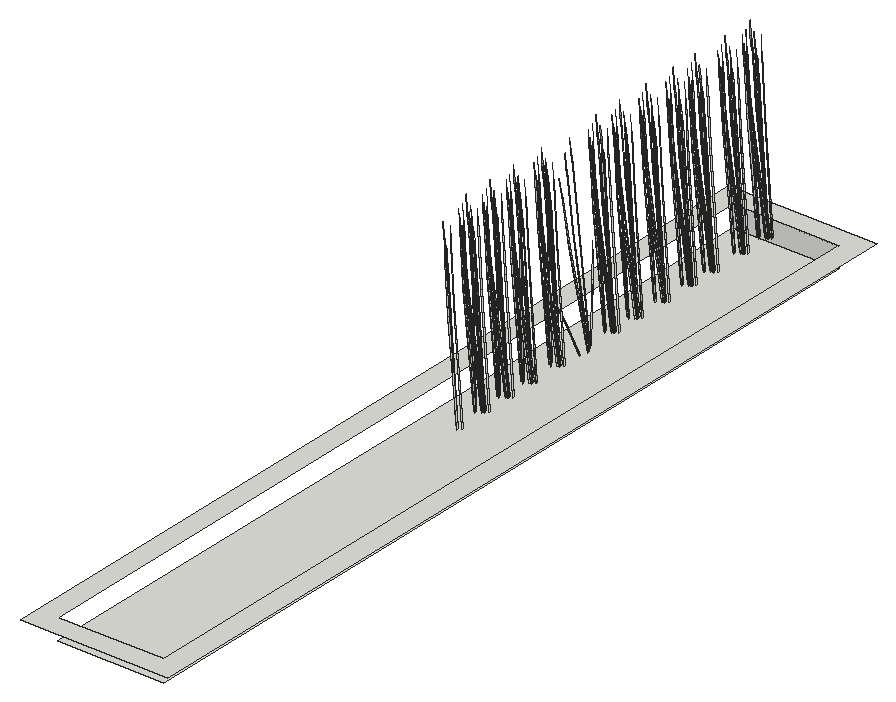
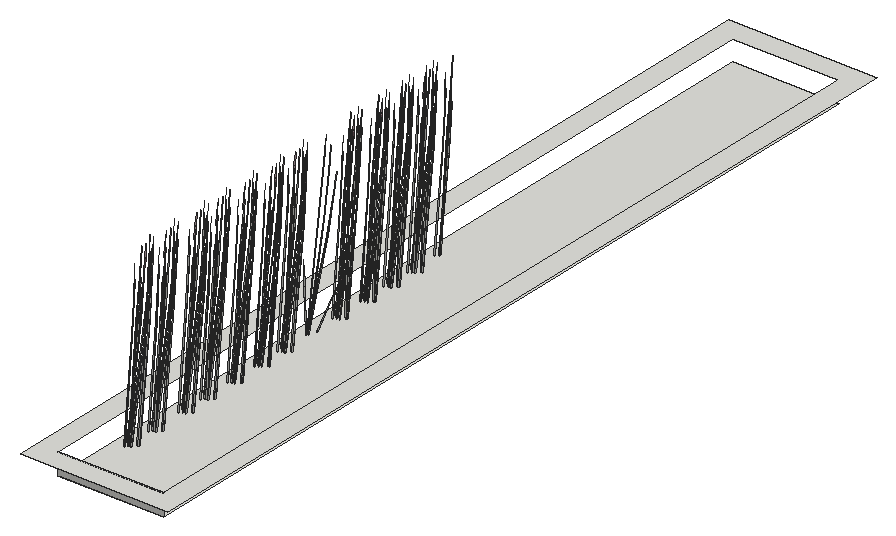
# SketchUp Ruby script. Lengths in inches.
U = 1.inch
M = Sketchup.active_model
def pt(a) = Geom::Point3d.new(a.map { |v| v * U })
def face(e, loops, mat)
  f = e.add_face(loops[0].map { |a| pt(a) })
  loops[1..].each { |l| e.add_face(l.map { |a| pt(a) }).erase! }
  f.material = f.back_material = mat if mat
  f
end
# faces: each face lists its corners as indices into pts; further lists are holes
def faces(e, pts, list, mat = nil) = list.each { |f| face(e, (f[0].is_a?(Array) ? f : [f]).map { |l| l.map { |i| pts[i] } }, mat) }
# xy, xz, yz: faces in a plane at the given z, y or x. An outline is a flat list of corners, or four numbers for a rectangle; further outlines are holes
def ring(l) = l.size == 4 ? [[l[0], l[1]], [l[2], l[1]], [l[2], l[3]], [l[0], l[3]]] : l.each_slice(2).to_a
def flat(e, list, mat, &to3) = list.each { |f| face(e, (f[0].is_a?(Array) ? f : [f]).map { |l| ring(l).map { |u, v| to3.(u, v) } }, mat) }
def xy(e, z, list, mat = nil) = flat(e, list, mat) { |x, y| [x, y, z] }
def xz(e, y, list, mat = nil) = flat(e, list, mat) { |x, z| [x, y, z] }
def yz(e, x, list, mat = nil) = flat(e, list, mat) { |y, z| [x, y, z] }
def lines(e, pts, list) = list.each { |a, b| e.add_line(pt(pts[a]), pt(pts[b])) }
# prism: a flat outline (further loops are holes) pulled along v
def prism(e, loops, v, mat = nil)
  f = face(e, loops, mat); d = Geom::Vector3d.new(v.map { |x| x * U })
  f.pushpull(f.normal.samedirection?(d) ? d.length : -d.length)
end
def box(e, o, s, mat = nil) = prism(e, [[o, [o[0] + s[0], o[1], o[2]], [o[0] + s[0], o[1] + s[1], o[2]], [o[0], o[1] + s[1], o[2]]]], [0, 0, s[2]], mat)
def at(x, y, z, deg = 0) = Geom::Transformation.translation(pt([x, y, z])) * Geom::Transformation.rotation(ORIGIN, Z_AXIS, deg.degrees)
def axes(o, x, y, z) = Geom::Transformation.new([*x, 0, *y, 0, *z, 0, *pt(o).to_a, 1])
def part(name) = M.definitions.add(name)
# library, detail: a bought-in or finely detailed component or shape, given as its bounding box
def library(name, o, s) = part(name).tap { |d| box(d.entities, o, s) }
def detail(e, o, s) = box(e.add_group.entities, o, s)
def put(e, d, t, mat = nil) = e.add_instance(d, t).tap { |i| i.material = mat if mat }
def group(e, t, mat = nil) = e.add_group.tap { |g| g.transformation = t; g.material = mat if mat }.entities
root = M.entities
M.materials.add("LightPink_Translucent").color = [144, 107, 117]
M.materials["LightPink_Translucent"].alpha = 0.75
c1 = part("blade")
p = [[2.15,0.21,22],[0,0.17,0],[0.09,0.45,0],[2.18,0.31,22],[2.29,0.31,22],[0.38,0.45,0],
  [2.48,0.24,33],[2.49,0.24,33],[2.48,0.22,33]]
faces(c1.entities,p,[[0,1,2,3],[4,5,2,3],[6,3,4,7],[8,0,3,6]])
c2 = part("seeds")
p = [[0.3,-0.1,1.38],[-0.01,-0.03,1.59],[-0.01,-0.03,0.03],[0.14,-0.07,-0.07],[0.29,-0.03,3],[0.15,0.01,3.11]]
faces(c2.entities,p,[[0,1,2,3],[1,0,4,5]],"LightPink_Translucent")
c3 = part("blade with seeds")
put(c3.entities,c1,at(0,0,0))
put(c3.entities,c2,axes([2.4,0.25,30.99],[1.5799,-0.05474,1.17369],[-0.12525,1.92788,0.29478],[-0.07173,-0.02425,1.56792]))
xy(root,42,[[316,268,346,508]])
xy(root,48,[[[310,262,352,514],[316,268,346,508]]])
xz(root,508,[[316,42,346,48]])
put(root,c3,axes([332.95,388.27,50.19],[0.47255,0.19538,0.43871],[-0.28245,0.35034,0],[-0.10763,-0.0445,1.3917]))
put(root,c3,axes([334,387.6,49.95],[-0.54829,0.02412,-0.39531],[-0.04958,-0.40041,0.19025],[-0.09816,0.04058,1.26923]))
put(root,c3,axes([334.02,387.83,49.82],[-0.34009,0.2937,-0.55095],[-0.42248,-0.26632,-0.1446],[-0.13628,0.07327,1.21613]))
put(root,c3,axes([334.58,388.63,49.78],[-0.47255,0.19538,-0.43871],[-0.28245,-0.35034,0],[-0.10763,0.0445,1.3917]))
put(root,c3,axes([331.78,396.37,49.78],[0,-0.39075,-0.43871],[0.56491,0,0],[0,-0.089,1.3917]))
put(root,c3,axes([331.64,396.66,50.1],[-0.63136,0,0],[0,-0.43672,-0.456],[0,-0.09947,1.44655]))
put(root,c3,axes([332.125,396.55,50.06],[-0.46965,0.32852,0.27176],[-0.46994,-0.32506,-0.32244],[-0.0164,-0.09329,1.45692]))
put(root,c3,axes([333.4,397.23,50.16],[0.13383,-0.46302,-0.20702],[0.63453,0.08071,0.45303],[-0.11087,-0.06394,1.38231]))
put(root,c3,axes([332.02,396.73,50.19],[0,0.39075,0.43871],[-0.56491,0,0],[0,-0.089,1.3917]))
put(root,c3,axes([333.35,397.05,49.95],[-0.30332,-0.32798,-0.39531],[0.45944,-0.23096,0.19025],[-0.09816,-0.04058,1.26923]))
put(root,c3,axes([332.52,397.77,49.79],[-0.11861,-0.34048,-0.27372],[0.47106,-0.09668,0.27372],[-0.09497,-0.03926,1.22797]))
put(root,c3,axes([333.63,397.34,50.3125],[-0.09741,0.34873,0.12794],[-0.4759,-0.06053,-0.36534],[-0.08661,-0.03581,1.11991]))
put(root,c3,axes([334.25,397.35,50.18],[-0.49304,-0.31451,-0.2226],[0.41487,-0.35316,0.48713],[-0.13277,0.03679,1.48635]))
put(root,c3,axes([332.95,397.95,50.19],[0.47255,0.19538,0.43871],[-0.28245,0.35034,0],[-0.10763,-0.0445,1.3917]))
put(root,c3,axes([334,397.28,49.95],[-0.54829,0.02412,-0.39531],[-0.04958,-0.40041,0.19025],[-0.09816,0.04058,1.26923]))
put(root,c3,axes([334.02,397.51,49.82],[-0.34009,0.2937,-0.55095],[-0.42248,-0.26632,-0.1446],[-0.13628,0.07327,1.21613]))
put(root,c3,axes([334.58,398.31,49.78],[-0.47255,0.19538,-0.43871],[-0.28245,-0.35034,0],[-0.10763,0.0445,1.3917]))
put(root,c3,axes([331.78,404.83,49.78],[0,-0.39075,-0.43871],[0.56491,0,0],[0,-0.089,1.3917]))
put(root,c3,axes([331.64,405.125,50.1],[-0.63136,0,0],[0,-0.43672,-0.456],[0,-0.09947,1.44655]))
put(root,c3,axes([332.125,405.01,50.06],[-0.46965,0.32852,0.27176],[-0.46994,-0.32506,-0.32244],[-0.0164,-0.09329,1.45692]))
put(root,c3,axes([333.4,405.7,50.16],[0.13383,-0.46302,-0.20702],[0.63453,0.08071,0.45303],[-0.11087,-0.06394,1.38231]))
put(root,c3,axes([332.02,405.19,50.19],[0,0.39075,0.43871],[-0.56491,0,0],[0,-0.089,1.3917]))
put(root,c3,axes([333.35,405.51,49.95],[-0.30332,-0.32798,-0.39531],[0.45944,-0.23096,0.19025],[-0.09816,-0.04058,1.26923]))
put(root,c3,axes([332.52,406.24,49.79],[-0.11861,-0.34048,-0.27372],[0.47106,-0.09668,0.27372],[-0.09497,-0.03926,1.22797]))
put(root,c3,axes([333.63,405.8,50.3125],[-0.09741,0.34873,0.12794],[-0.4759,-0.06053,-0.36534],[-0.08661,-0.03581,1.11991]))
put(root,c3,axes([334.25,405.81,50.18],[-0.49304,-0.31451,-0.2226],[0.41487,-0.35316,0.48713],[-0.13277,0.03679,1.48635]))
put(root,c3,axes([332.95,406.41,50.19],[0.47255,0.19538,0.43871],[-0.28245,0.35034,0],[-0.10763,-0.0445,1.3917]))
put(root,c3,axes([334,405.74,49.95],[-0.54829,0.02412,-0.39531],[-0.04958,-0.40041,0.19025],[-0.09816,0.04058,1.26923]))
put(root,c3,axes([334.02,405.97,49.82],[-0.34009,0.2937,-0.55095],[-0.42248,-0.26632,-0.1446],[-0.13628,0.07327,1.21613]))
put(root,c3,axes([334.58,406.78,49.78],[-0.47255,0.19538,-0.43871],[-0.28245,-0.35034,0],[-0.10763,0.0445,1.3917]))
put(root,c3,axes([331.78,413.3,49.78],[0,-0.39075,-0.43871],[0.56491,0,0],[0,-0.089,1.3917]))
put(root,c3,axes([331.64,413.59,50.1],[-0.63136,0,0],[0,-0.43672,-0.456],[0,-0.09947,1.44655]))
put(root,c3,axes([332.125,413.48,50.06],[-0.46965,0.32852,0.27176],[-0.46994,-0.32506,-0.32244],[-0.0164,-0.09329,1.45692]))
put(root,c3,axes([333.4,414.16,50.16],[0.13383,-0.46302,-0.20702],[0.63453,0.08071,0.45303],[-0.11087,-0.06394,1.38231]))
put(root,c3,axes([332.02,413.66,50.19],[0,0.39075,0.43871],[-0.56491,0,0],[0,-0.089,1.3917]))
put(root,c3,axes([333.35,413.97,49.95],[-0.30332,-0.32798,-0.39531],[0.45944,-0.23096,0.19025],[-0.09816,-0.04058,1.26923]))
put(root,c3,axes([332.52,414.7,49.79],[-0.11861,-0.34048,-0.27372],[0.47106,-0.09668,0.27372],[-0.09497,-0.03926,1.22797]))
put(root,c3,axes([333.63,414.27,50.3125],[-0.09741,0.34873,0.12794],[-0.4759,-0.06053,-0.36534],[-0.08661,-0.03581,1.11991]))
put(root,c3,axes([334.25,414.28,50.18],[-0.49304,-0.31451,-0.2226],[0.41487,-0.35316,0.48713],[-0.13277,0.03679,1.48635]))
put(root,c3,axes([332.95,414.88,50.19],[0.47255,0.19538,0.43871],[-0.28245,0.35034,0],[-0.10763,-0.0445,1.3917]))
put(root,c3,axes([334,414.21,49.95],[-0.54829,0.02412,-0.39531],[-0.04958,-0.40041,0.19025],[-0.09816,0.04058,1.26923]))
put(root,c3,axes([334.02,414.44,49.82],[-0.34009,0.2937,-0.55095],[-0.42248,-0.26632,-0.1446],[-0.13628,0.07327,1.21613]))
put(root,c3,axes([334.58,415.24,49.78],[-0.47255,0.19538,-0.43871],[-0.28245,-0.35034,0],[-0.10763,0.0445,1.3917]))
put(root,c3,axes([331.78,423.19,49.78],[0,-0.39075,-0.43871],[0.56491,0,0],[0,-0.089,1.3917]))
put(root,c3,axes([331.64,423.49,50.1],[-0.63136,0,0],[0,-0.43672,-0.456],[0,-0.09947,1.44655]))
put(root,c3,axes([332.125,423.375,50.06],[-0.46965,0.32852,0.27176],[-0.46994,-0.32506,-0.32244],[-0.0164,-0.09329,1.45692]))
put(root,c3,axes([333.4,424.06,50.16],[0.13383,-0.46302,-0.20702],[0.63453,0.08071,0.45303],[-0.11087,-0.06394,1.38231]))
put(root,c3,axes([332.02,423.56,50.19],[0,0.39075,0.43871],[-0.56491,0,0],[0,-0.089,1.3917]))
put(root,c3,axes([333.35,423.87,49.95],[-0.30332,-0.32798,-0.39531],[0.45944,-0.23096,0.19025],[-0.09816,-0.04058,1.26923]))
put(root,c3,axes([332.52,424.6,49.79],[-0.11861,-0.34048,-0.27372],[0.47106,-0.09668,0.27372],[-0.09497,-0.03926,1.22797]))
put(root,c3,axes([333.63,424.17,50.3125],[-0.09741,0.34873,0.12794],[-0.4759,-0.06053,-0.36534],[-0.08661,-0.03581,1.11991]))
put(root,c3,axes([334.25,424.17,50.18],[-0.49304,-0.31451,-0.2226],[0.41487,-0.35316,0.48713],[-0.13277,0.03679,1.48635]))
put(root,c3,axes([332.95,424.78,50.19],[0.47255,0.19538,0.43871],[-0.28245,0.35034,0],[-0.10763,-0.0445,1.3917]))
put(root,c3,axes([334,424.11,49.95],[-0.54829,0.02412,-0.39531],[-0.04958,-0.40041,0.19025],[-0.09816,0.04058,1.26923]))
put(root,c3,axes([334.02,424.34,49.82],[-0.34009,0.2937,-0.55095],[-0.42248,-0.26632,-0.1446],[-0.13628,0.07327,1.21613]))
put(root,c3,axes([334.58,425.14,49.78],[-0.47255,0.19538,-0.43871],[-0.28245,-0.35034,0],[-0.10763,0.0445,1.3917]))
put(root,c3,axes([333.77,431.35,49.32],[-0.04891,0.05148,1.55816],[-0.49427,0.11098,-0.23804],[-0.1194,-0.10096,0.26541]))
put(root,c3,axes([334.67,433.52,49.82],[-0.52523,-0.06406,-0.55095],[0.11084,-0.39517,-0.1446],[-0.15674,-0.04788,1.21613]))
put(root,c3,axes([333.98,434.26,49.78],[-0.47255,-0.19538,-0.43871],[0.28245,-0.35034,0],[-0.10763,-0.0445,1.3917]))
put(root,c3,axes([334.27,434.5,50.1],[-0.31568,0.39156,0],[-0.52815,-0.21836,-0.456],[-0.12029,-0.04973,1.44655]))
put(root,c3,axes([333.69,435.07,50.29],[0.15933,-0.06164,1.26356],[0.39339,0.18587,-0.27174],[-0.11709,0.16083,0.54024]))
put(root,c3,axes([331.78,442.58,49.78],[0,-0.39075,-0.43871],[0.56491,0,0],[0,-0.089,1.3917]))
put(root,c3,axes([331.64,442.875,50.1],[-0.63136,0,0],[0,-0.43672,-0.456],[0,-0.09947,1.44655]))
put(root,c3,axes([332.125,442.76,50.06],[-0.46965,0.32852,0.27176],[-0.46994,-0.32506,-0.32244],[-0.0164,-0.09329,1.45692]))
put(root,c3,axes([333.4,443.44,50.16],[0.13383,-0.46302,-0.20702],[0.63453,0.08071,0.45303],[-0.11087,-0.06394,1.38231]))
put(root,c3,axes([333.35,443.26,49.95],[-0.30332,-0.32798,-0.39531],[0.45944,-0.23096,0.19025],[-0.09816,-0.04058,1.26923]))
put(root,c3,axes([332.52,443.98,49.79],[-0.11861,-0.34048,-0.27372],[0.47106,-0.09668,0.27372],[-0.09497,-0.03926,1.22797]))
put(root,c3,axes([333.63,443.55,50.3125],[-0.09741,0.34873,0.12794],[-0.4759,-0.06053,-0.36534],[-0.08661,-0.03581,1.11991]))
put(root,c3,axes([334.25,443.56,50.18],[-0.49304,-0.31451,-0.2226],[0.41487,-0.35316,0.48713],[-0.13277,0.03679,1.48635]))
put(root,c3,axes([332.95,444.16,50.19],[0.47255,0.19538,0.43871],[-0.28245,0.35034,0],[-0.10763,-0.0445,1.3917]))
put(root,c3,axes([334,443.49,49.95],[-0.54829,0.02412,-0.39531],[-0.04958,-0.40041,0.19025],[-0.09816,0.04058,1.26923]))
put(root,c3,axes([334.02,443.72,49.82],[-0.34009,0.2937,-0.55095],[-0.42248,-0.26632,-0.1446],[-0.13628,0.07327,1.21613]))
put(root,c3,axes([334.58,444.53,49.78],[-0.47255,0.19538,-0.43871],[-0.28245,-0.35034,0],[-0.10763,0.0445,1.3917]))
put(root,c3,axes([331.78,450.95,49.78],[0,-0.39075,-0.43871],[0.56491,0,0],[0,-0.089,1.3917]))
put(root,c3,axes([331.64,451.25,50.1],[-0.63136,0,0],[0,-0.43672,-0.456],[0,-0.09947,1.44655]))
put(root,c3,axes([332.125,451.13,50.06],[-0.46965,0.32852,0.27176],[-0.46994,-0.32506,-0.32244],[-0.0164,-0.09329,1.45692]))
put(root,c3,axes([333.4,451.82,50.16],[0.13383,-0.46302,-0.20702],[0.63453,0.08071,0.45303],[-0.11087,-0.06394,1.38231]))
put(root,c3,axes([333.35,451.63,49.95],[-0.30332,-0.32798,-0.39531],[0.45944,-0.23096,0.19025],[-0.09816,-0.04058,1.26923]))
put(root,c3,axes([332.52,452.36,49.79],[-0.11861,-0.34048,-0.27372],[0.47106,-0.09668,0.27372],[-0.09497,-0.03926,1.22797]))
put(root,c3,axes([333.63,451.93,50.3125],[-0.09741,0.34873,0.12794],[-0.4759,-0.06053,-0.36534],[-0.08661,-0.03581,1.11991]))
put(root,c3,axes([334.25,451.93,50.18],[-0.49304,-0.31451,-0.2226],[0.41487,-0.35316,0.48713],[-0.13277,0.03679,1.48635]))
put(root,c3,axes([332.95,452.53,50.19],[0.47255,0.19538,0.43871],[-0.28245,0.35034,0],[-0.10763,-0.0445,1.3917]))
put(root,c3,axes([334,451.86,49.95],[-0.54829,0.02412,-0.39531],[-0.04958,-0.40041,0.19025],[-0.09816,0.04058,1.26923]))
put(root,c3,axes([334.02,452.1,49.82],[-0.34009,0.2937,-0.55095],[-0.42248,-0.26632,-0.1446],[-0.13628,0.07327,1.21613]))
put(root,c3,axes([334.58,452.9,49.78],[-0.47255,0.19538,-0.43871],[-0.28245,-0.35034,0],[-0.10763,0.0445,1.3917]))
put(root,c3,axes([331.78,460.47,49.78],[0,-0.39075,-0.43871],[0.56491,0,0],[0,-0.089,1.3917]))
put(root,c3,axes([331.64,460.76,50.1],[-0.63136,0,0],[0,-0.43672,-0.456],[0,-0.09947,1.44655]))
put(root,c3,axes([332.125,460.65,50.06],[-0.46965,0.32852,0.27176],[-0.46994,-0.32506,-0.32244],[-0.0164,-0.09329,1.45692]))
put(root,c3,axes([333.4,461.33,50.16],[0.13383,-0.46302,-0.20702],[0.63453,0.08071,0.45303],[-0.11087,-0.06394,1.38231]))
put(root,c3,axes([333.35,461.14,49.95],[-0.30332,-0.32798,-0.39531],[0.45944,-0.23096,0.19025],[-0.09816,-0.04058,1.26923]))
put(root,c3,axes([332.52,461.87,49.79],[-0.11861,-0.34048,-0.27372],[0.47106,-0.09668,0.27372],[-0.09497,-0.03926,1.22797]))
put(root,c3,axes([333.63,461.44,50.3125],[-0.09741,0.34873,0.12794],[-0.4759,-0.06053,-0.36534],[-0.08661,-0.03581,1.11991]))
put(root,c3,axes([334.25,461.45,50.18],[-0.49304,-0.31451,-0.2226],[0.41487,-0.35316,0.48713],[-0.13277,0.03679,1.48635]))
put(root,c3,axes([332.95,462.05,50.19],[0.47255,0.19538,0.43871],[-0.28245,0.35034,0],[-0.10763,-0.0445,1.3917]))
put(root,c3,axes([334,461.38,49.95],[-0.54829,0.02412,-0.39531],[-0.04958,-0.40041,0.19025],[-0.09816,0.04058,1.26923]))
put(root,c3,axes([334.02,461.61,49.82],[-0.34009,0.2937,-0.55095],[-0.42248,-0.26632,-0.1446],[-0.13628,0.07327,1.21613]))
put(root,c3,axes([334.58,462.41,49.78],[-0.47255,0.19538,-0.43871],[-0.28245,-0.35034,0],[-0.10763,0.0445,1.3917]))
put(root,c3,axes([331.78,470.02,49.78],[0,-0.39075,-0.43871],[0.56491,0,0],[0,-0.089,1.3917]))
put(root,c3,axes([331.64,470.32,50.1],[-0.63136,0,0],[0,-0.43672,-0.456],[0,-0.09947,1.44655]))
put(root,c3,axes([332.125,470.2,50.06],[-0.46965,0.32852,0.27176],[-0.46994,-0.32506,-0.32244],[-0.0164,-0.09329,1.45692]))
put(root,c3,axes([333.4,470.89,50.16],[0.13383,-0.46302,-0.20702],[0.63453,0.08071,0.45303],[-0.11087,-0.06394,1.38231]))
put(root,c3,axes([333.35,470.7,49.95],[-0.30332,-0.32798,-0.39531],[0.45944,-0.23096,0.19025],[-0.09816,-0.04058,1.26923]))
put(root,c3,axes([332.52,471.43,49.79],[-0.11861,-0.34048,-0.27372],[0.47106,-0.09668,0.27372],[-0.09497,-0.03926,1.22797]))
put(root,c3,axes([333.63,471,50.3125],[-0.09741,0.34873,0.12794],[-0.4759,-0.06053,-0.36534],[-0.08661,-0.03581,1.11991]))
put(root,c3,axes([334.25,471,50.18],[-0.49304,-0.31451,-0.2226],[0.41487,-0.35316,0.48713],[-0.13277,0.03679,1.48635]))
put(root,c3,axes([332.95,471.6,50.19],[0.47255,0.19538,0.43871],[-0.28245,0.35034,0],[-0.10763,-0.0445,1.3917]))
put(root,c3,axes([334,470.94,49.95],[-0.54829,0.02412,-0.39531],[-0.04958,-0.40041,0.19025],[-0.09816,0.04058,1.26923]))
put(root,c3,axes([334.02,471.17,49.82],[-0.34009,0.2937,-0.55095],[-0.42248,-0.26632,-0.1446],[-0.13628,0.07327,1.21613]))
put(root,c3,axes([334.58,471.97,49.78],[-0.47255,0.19538,-0.43871],[-0.28245,-0.35034,0],[-0.10763,0.0445,1.3917]))
put(root,c3,axes([331.78,477.82,49.78],[0,-0.39075,-0.43871],[0.56491,0,0],[0,-0.089,1.3917]))
put(root,c3,axes([331.64,478.11,50.1],[-0.63136,0,0],[0,-0.43672,-0.456],[0,-0.09947,1.44655]))
put(root,c3,axes([332.125,478,50.06],[-0.46965,0.32852,0.27176],[-0.46994,-0.32506,-0.32244],[-0.0164,-0.09329,1.45692]))
put(root,c3,axes([333.4,478.68,50.16],[0.13383,-0.46302,-0.20702],[0.63453,0.08071,0.45303],[-0.11087,-0.06394,1.38231]))
put(root,c3,axes([333.35,478.5,49.95],[-0.30332,-0.32798,-0.39531],[0.45944,-0.23096,0.19025],[-0.09816,-0.04058,1.26923]))
put(root,c3,axes([332.52,479.22,49.79],[-0.11861,-0.34048,-0.27372],[0.47106,-0.09668,0.27372],[-0.09497,-0.03926,1.22797]))
put(root,c3,axes([333.63,478.79,50.3125],[-0.09741,0.34873,0.12794],[-0.4759,-0.06053,-0.36534],[-0.08661,-0.03581,1.11991]))
put(root,c3,axes([334.25,478.8,50.18],[-0.49304,-0.31451,-0.2226],[0.41487,-0.35316,0.48713],[-0.13277,0.03679,1.48635]))
put(root,c3,axes([332.95,479.4,50.19],[0.47255,0.19538,0.43871],[-0.28245,0.35034,0],[-0.10763,-0.0445,1.3917]))
put(root,c3,axes([334,478.73,49.95],[-0.54829,0.02412,-0.39531],[-0.04958,-0.40041,0.19025],[-0.09816,0.04058,1.26923]))
put(root,c3,axes([334.02,478.96,49.82],[-0.34009,0.2937,-0.55095],[-0.42248,-0.26632,-0.1446],[-0.13628,0.07327,1.21613]))
put(root,c3,axes([334.58,479.77,49.78],[-0.47255,0.19538,-0.43871],[-0.28245,-0.35034,0],[-0.10763,0.0445,1.3917]))
put(root,c3,axes([331.78,488.52,49.78],[0,-0.39075,-0.43871],[0.56491,0,0],[0,-0.089,1.3917]))
put(root,c3,axes([331.64,488.81,50.1],[-0.63136,0,0],[0,-0.43672,-0.456],[0,-0.09947,1.44655]))
put(root,c3,axes([332.125,488.7,50.06],[-0.46965,0.32852,0.27176],[-0.46994,-0.32506,-0.32244],[-0.0164,-0.09329,1.45692]))
put(root,c3,axes([333.4,489.38,50.16],[0.13383,-0.46302,-0.20702],[0.63453,0.08071,0.45303],[-0.11087,-0.06394,1.38231]))
put(root,c3,axes([333.35,489.2,49.95],[-0.30332,-0.32798,-0.39531],[0.45944,-0.23096,0.19025],[-0.09816,-0.04058,1.26923]))
put(root,c3,axes([332.52,489.92,49.79],[-0.11861,-0.34048,-0.27372],[0.47106,-0.09668,0.27372],[-0.09497,-0.03926,1.22797]))
put(root,c3,axes([333.63,489.49,50.3125],[-0.09741,0.34873,0.12794],[-0.4759,-0.06053,-0.36534],[-0.08661,-0.03581,1.11991]))
put(root,c3,axes([334.25,489.5,50.18],[-0.49304,-0.31451,-0.2226],[0.41487,-0.35316,0.48713],[-0.13277,0.03679,1.48635]))
put(root,c3,axes([332.95,490.1,50.19],[0.47255,0.19538,0.43871],[-0.28245,0.35034,0],[-0.10763,-0.0445,1.3917]))
put(root,c3,axes([334,489.43,49.95],[-0.54829,0.02412,-0.39531],[-0.04958,-0.40041,0.19025],[-0.09816,0.04058,1.26923]))
put(root,c3,axes([334.02,489.66,49.82],[-0.34009,0.2937,-0.55095],[-0.42248,-0.26632,-0.1446],[-0.13628,0.07327,1.21613]))
put(root,c3,axes([334.58,490.47,49.78],[-0.47255,0.19538,-0.43871],[-0.28245,-0.35034,0],[-0.10763,0.0445,1.3917]))
put(root,c3,axes([331.78,497.3,49.78],[0,-0.39075,-0.43871],[0.56491,0,0],[0,-0.089,1.3917]))
put(root,c3,axes([331.64,497.59,50.1],[-0.63136,0,0],[0,-0.43672,-0.456],[0,-0.09947,1.44655]))
put(root,c3,axes([332.125,497.48,50.06],[-0.46965,0.32852,0.27176],[-0.46994,-0.32506,-0.32244],[-0.0164,-0.09329,1.45692]))
put(root,c3,axes([333.4,498.16,50.16],[0.13383,-0.46302,-0.20702],[0.63453,0.08071,0.45303],[-0.11087,-0.06394,1.38231]))
put(root,c3,axes([333.35,497.97,49.95],[-0.30332,-0.32798,-0.39531],[0.45944,-0.23096,0.19025],[-0.09816,-0.04058,1.26923]))
put(root,c3,axes([332.52,498.7,49.79],[-0.11861,-0.34048,-0.27372],[0.47106,-0.09668,0.27372],[-0.09497,-0.03926,1.22797]))
put(root,c3,axes([333.63,498.27,50.3125],[-0.09741,0.34873,0.12794],[-0.4759,-0.06053,-0.36534],[-0.08661,-0.03581,1.11991]))
put(root,c3,axes([334.25,498.28,50.18],[-0.49304,-0.31451,-0.2226],[0.41487,-0.35316,0.48713],[-0.13277,0.03679,1.48635]))
put(root,c3,axes([332.95,498.88,50.19],[0.47255,0.19538,0.43871],[-0.28245,0.35034,0],[-0.10763,-0.0445,1.3917]))
put(root,c3,axes([334,498.21,49.95],[-0.54829,0.02412,-0.39531],[-0.04958,-0.40041,0.19025],[-0.09816,0.04058,1.26923]))
put(root,c3,axes([334.02,498.44,49.82],[-0.34009,0.2937,-0.55095],[-0.42248,-0.26632,-0.1446],[-0.13628,0.07327,1.21613]))
put(root,c3,axes([334.58,499.24,49.78],[-0.47255,0.19538,-0.43871],[-0.28245,-0.35034,0],[-0.10763,0.0445,1.3917]))
